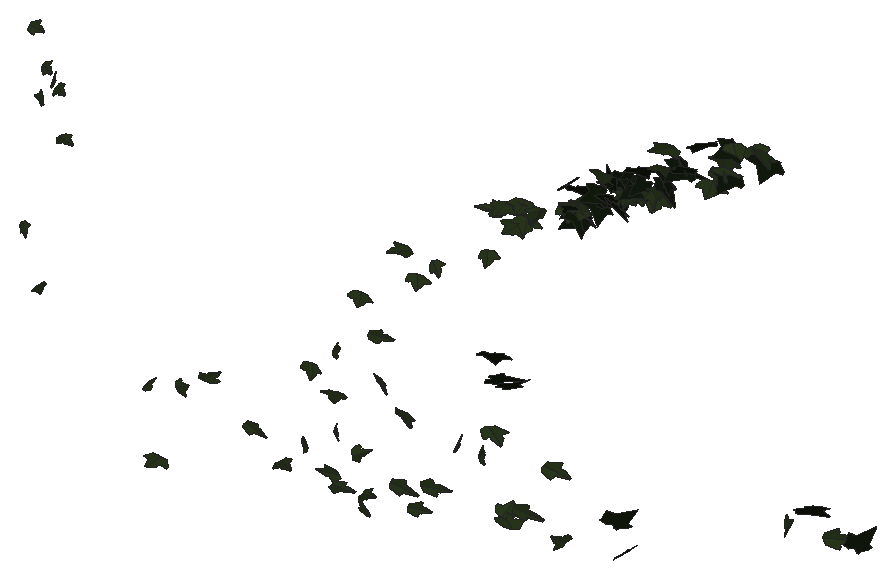
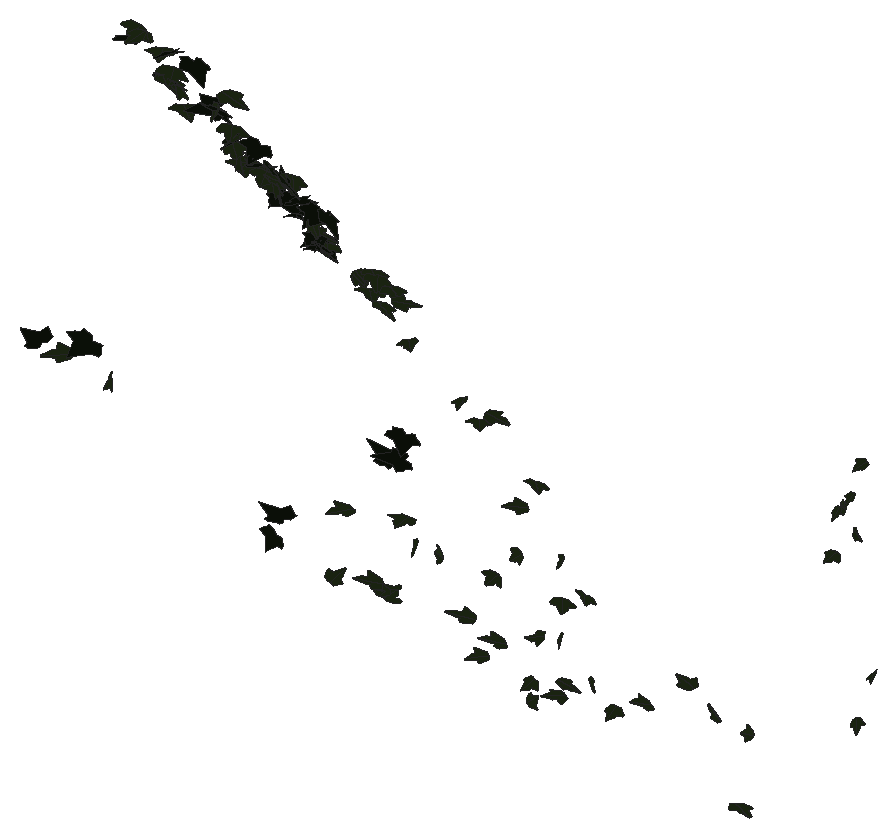
# SketchUp Ruby script. Lengths in millimetres.
U = 1.mm
M = Sketchup.active_model
def pt(a) = Geom::Point3d.new(a.map { |v| v * U })
def face(e, loops, mat)
  f = e.add_face(loops[0].map { |a| pt(a) })
  loops[1..].each { |l| e.add_face(l.map { |a| pt(a) }).erase! }
  f.material = f.back_material = mat if mat
  f
end
# faces: each face lists its corners as indices into pts; further lists are holes
def faces(e, pts, list, mat = nil) = list.each { |f| face(e, (f[0].is_a?(Array) ? f : [f]).map { |l| l.map { |i| pts[i] } }, mat) }
# xy, xz, yz: faces in a plane at the given z, y or x. An outline is a flat list of corners, or four numbers for a rectangle; further outlines are holes
def ring(l) = l.size == 4 ? [[l[0], l[1]], [l[2], l[1]], [l[2], l[3]], [l[0], l[3]]] : l.each_slice(2).to_a
def flat(e, list, mat, &to3) = list.each { |f| face(e, (f[0].is_a?(Array) ? f : [f]).map { |l| ring(l).map { |u, v| to3.(u, v) } }, mat) }
def xy(e, z, list, mat = nil) = flat(e, list, mat) { |x, y| [x, y, z] }
def xz(e, y, list, mat = nil) = flat(e, list, mat) { |x, z| [x, y, z] }
def yz(e, x, list, mat = nil) = flat(e, list, mat) { |y, z| [x, y, z] }
def lines(e, pts, list) = list.each { |a, b| e.add_line(pt(pts[a]), pt(pts[b])) }
# prism: a flat outline (further loops are holes) pulled along v
def prism(e, loops, v, mat = nil)
  f = face(e, loops, mat); d = Geom::Vector3d.new(v.map { |x| x * U })
  f.pushpull(f.normal.samedirection?(d) ? d.length : -d.length)
end
def box(e, o, s, mat = nil) = prism(e, [[o, [o[0] + s[0], o[1], o[2]], [o[0] + s[0], o[1] + s[1], o[2]], [o[0], o[1] + s[1], o[2]]]], [0, 0, s[2]], mat)
def at(x, y, z, deg = 0) = Geom::Transformation.translation(pt([x, y, z])) * Geom::Transformation.rotation(ORIGIN, Z_AXIS, deg.degrees)
def axes(o, x, y, z) = Geom::Transformation.new([*x, 0, *y, 0, *z, 0, *pt(o).to_a, 1])
def part(name) = M.definitions.add(name)
# library, detail: a bought-in or finely detailed component or shape, given as its bounding box
def library(name, o, s) = part(name).tap { |d| box(d.entities, o, s) }
def detail(e, o, s) = box(e.add_group.entities, o, s)
def put(e, d, t, mat = nil) = e.add_instance(d, t).tap { |i| i.material = mat if mat }
def group(e, t, mat = nil) = e.add_group.tap { |g| g.transformation = t; g.material = mat if mat }.entities
root = M.entities
M.materials.add("efeu1").color = [18, 25, 13]
M.materials.add("efeu2").color = [43, 57, 29]
c1 = part("ivyleaf_10")
p = [[0,12.8,-0.8],[-1.5,51.3,-10.9],[-4.9,51,-11.6],[-13.6,26.5,-7.3],[-13.2,15.9,-4.6],[-21.1,19.3,-7.2],
  [-29.5,16.3,-8.3],[-29.2,8.3,-6.2],[-19.7,-9.8,0.5],[-7.6,-13,4],[1,-12.2,5.8],[-0.4,51.1,-11.1],
  [-1.5,51.1,-10.9],[1,-12.4,5.9],[16.9,-12.4,3.5],[35.1,9.1,-5.1],[35,12.9,-6.1],[20.5,16.4,-4.9],
  [15.8,15,-3.8],[15.3,27.6,-7.1],[12.8,31.3,-7.8]]
faces(c1.entities,p,[[0,1,2,3,4,5,6,7,8,9,10],[11,12,0,13,14,15,16,17,18,19,20]],"efeu2")
c2 = part("ivyleaf_9")
p = [[39.1,54.8,31.7],[34.5,51.8,30.2],[-5.3,25.2,17.3],[-17.9,28.3,20.9],[-21.6,21.7,17],[-20.2,4.3,5.3],
  [-22.9,-0.3,2.5],[-17.1,-4,-0.6],[-2,-2.1,-1.2],[-0.7,-15.4,-10.1],[16.6,-22.3,-16.7],[21.1,-15.1,-12.5],
  [32.7,-10.7,-11],[46.1,-1.8,-6.6],[30.8,11.2,3.8]]
faces(c2.entities,p,[[0,1,2,3,4,5,6,7,8,9,10,11,12,13,14]],"efeu1")
put(root,c1,axes([1835,1080.9,259.8],[0.07,0.0363,-0.75049],[0.72421,0.647,0.04994],[1.23306,-0.38207,0.01327]))
put(root,c1,axes([716.7,1092.8,545.6],[-0.03211,0.64084,-0.00687],[0.00479,-0.00671,-0.64137],[-0.78186,-0.02636,-0.00365]))
put(root,c1,axes([1134.4,1084.8,213.7],[0.18479,-0.3198,0.55072],[-0.13417,0.54826,0.3308],[-1.20458,-0.11013,0.04764]))
put(root,c1,axes([755.1,1084.5,1157.1],[0.17773,0.33378,0.55382],[0.19747,0.5308,-0.36249],[-0.76376,0.21491,0.03515]))
put(root,c1,axes([772,1093.8,384.4],[-0.22942,-0.59673,-0.12491],[0.01796,0.12623,-0.62522],[0.74357,-0.18716,-0.02343]))
put(root,c1,axes([850,1090.9,855.9],[-0.51761,-0.26028,-0.40786],[0.44142,0.18947,-0.49728],[0.3919,-0.55719,0.02142]))
put(root,c1,axes([815.9,1090.9,1003.2],[0.31464,-0.47607,0.34173],[-0.21038,0.29518,0.54136],[-0.68329,-0.3101,-0.00932]))
put(root,c1,axes([779.9,1090.9,945],[-0.08194,0.1069,0.6259],[-0.73806,0.18038,-0.09572],[-0.23526,-0.60309,0.08231]))
put(root,c1,axes([793.1,1087.6,1049],[0.02924,0.51162,0.38768],[-0.04677,0.3884,-0.5102],[-0.78173,-0.00411,0.04503]))
put(root,c1,axes([2260.2,1098.7,999.9],[0.65638,0.60263,-0.13044],[-0.19629,-0.09097,-0.69297],[-1.15696,0.35733,0.04357]))
put(root,c1,axes([1958.8,1094.8,204.7],[0.29609,0.07308,0.70938],[1.27007,0.2411,-0.17119],[-0.47857,0.68505,-0.01543]))
put(root,c1,axes([1227.7,1103.9,237.8],[0.58443,-0.30845,-0.46453],[0.60756,-0.33756,0.43517],[-0.87012,-0.44287,-0.00815]))
put(root,c1,axes([2065.8,1090.3,238.7],[-0.15506,-0.04365,0.74271],[1.07084,0.48522,0.09024],[-0.92642,0.56817,-0.02]))
put(root,c1,axes([1888.8,1090.1,630.5],[0.22873,0.00111,0.64955],[0.80459,0.50138,-0.07907],[-0.93855,0.43009,0.09051]))
put(root,c1,axes([1833.4,1100.7,725.7],[1.20506,0.07836,-0.00643],[-0.01143,-0.00382,-0.638],[-0.1492,0.6332,-0.00305]))
put(root,c1,axes([2161.9,1090.9,387.6],[0.43544,-0.49458,0.48892],[-0.33564,0.45661,0.54443],[-1.28032,-0.28791,0.02356]))
put(root,c1,axes([832.1,1095.1,997],[-0.12067,-0.54731,-0.31172],[0.27731,0.26326,-0.53435],[0.71664,-0.19403,0.15429]))
put(root,c1,axes([2022.3,1099.8,844.8],[0.99723,0.41506,-0.01188],[-0.01976,-0.00603,-0.66845],[-0.79003,0.52408,0.00172]))
put(root,c1,axes([1157.7,1102.7,-0.6],[1.01432,0.16087,-0.33534],[-0.61084,-0.09718,-0.55671],[-0.3577,0.62214,-0.00025]))
put(root,c2,axes([2278.7,1091.8,709.9],[0.96894,0.53705,-0.1811],[-0.23679,-0.1316,-0.74001],[-1.05235,0.52409,-0.00024]))
put(root,c2,axes([2681.3,1095.3,1297.3],[1.34853,-0.13217,-0.26729],[-0.50396,0.03793,-0.72071],[0.26093,0.75635,-0.01057]))
put(root,c1,axes([1324.2,1097.1,299.3],[-0.61086,-0.43006,0.38361],[0.44145,0.30555,0.53663],[-1.00403,0.396,0.00255]))
put(root,c1,axes([1578.7,1095.4,139],[-0.5423,-0.5139,-0.37911],[0.42223,0.30962,-0.58645],[1.13969,-0.35924,0.03688]))
put(root,c1,axes([3165.4,1100.4,1618.4],[-1.49985,0.25492,-0.22503],[0.39022,-0.0969,-0.8278],[-0.51628,-0.81382,0.02807]))
put(root,c1,axes([1749.5,1101.1,402.9],[-1.12343,-0.23675,0.0375],[-0.06558,-0.01482,-0.63599],[0.45147,-0.59129,0.00093]))
put(root,c1,axes([2864.2,1103.2,1524.3],[0.82011,0.30587,-0.61086],[-1.25968,0.00806,-0.46287],[-0.32199,0.74751,0.25495]))
put(root,c2,axes([2319.3,1098.5,624.8],[0.92747,0.59527,-0.0229],[0.02688,0.01804,0.7693],[1.13344,-0.48753,0.0005]))
put(root,c1,axes([1746.8,1100.9,162.2],[0.3893,-0.06424,-0.6006],[-1.0995,0.16432,-0.21433],[0.33562,0.61283,-0.00548]))
put(root,c2,axes([3330.2,1087,617.3],[1.21286,0.57336,0.31985],[0.44231,0.21988,-0.85721],[-1.16862,0.67829,0.00751]))
put(root,c1,axes([1891.6,1104.2,494.7],[-0.79385,0.48435,-0.28142],[0.34691,-0.21441,-0.6392],[-1.00809,-0.4552,0.00164]))
put(root,c2,axes([2979,1097.4,1579.8],[0.19677,0.7596,-0.27697],[-0.16077,-0.26755,-0.76529],[-1.53035,0.12577,0.04479]))
put(root,c2,axes([3495.2,1090.6,562.5],[-0.38146,-0.14482,0.9022],[1.41128,0.51393,0.24723],[-1.01616,0.76812,0.00468]))
put(root,c1,axes([1663.6,1106.5,450.6],[1.15689,-0.18495,0.17352],[0.31226,-0.05682,-0.63535],[0.36803,0.62959,-0.00637]))
put(root,c1,axes([2245.2,1089.9,393.7],[-0.18723,0.20672,0.71004],[-0.61655,0.63187,-0.22884],[-1.26523,-0.3385,0.00644]))
put(root,c2,axes([3186.2,1116.5,1593.2],[-0.91707,-0.70197,0.06417],[-0.04945,-0.05998,-0.85134],[1.34064,-0.48239,0.01249]))
put(root,c1,axes([1757.9,1094,292.1],[-0.36104,0.3296,0.51373],[-0.51729,0.43607,-0.38014],[-1.04013,-0.33128,0.01074]))
put(root,c2,axes([3066.2,1121.5,1582.5],[-0.81268,-0.41233,0.56307],[-0.59755,-0.47604,-0.5867],[1.18624,-0.52228,0.09022]))
put(root,c2,axes([2629.2,1120.1,1296.5],[-0.82056,-0.40163,0.52611],[-0.73852,-0.35528,-0.58922],[1.02051,-0.58005,-0.00338]))
put(root,c1,axes([2330.3,1105.3,214.2],[1.22161,0.264,0.30917],[-0.54691,-0.11409,0.69403],[0.54732,-0.70325,0.00347]))
put(root,c2,axes([3060.3,1115.4,1509.6],[-1.47464,-0.18215,-0.25497],[0.51451,-0.04472,-0.78959],[0.30154,-0.81447,0.10037]))
put(root,c1,axes([2498.2,1119.5,213.9],[-0.43074,-0.39702,-0.64952],[-0.61961,-0.56204,0.45699],[-1.30963,0.39649,-0.00258]))
put(root,c1,axes([1458.8,1106.5,200.9],[0.47718,-0.00362,0.59161],[1.11,0.10933,-0.24651],[-0.18894,0.63317,0.04594]))
put(root,c2,axes([2616,1118.7,1265.3],[-0.50362,-0.7383,0.0523],[0.05061,-0.06499,-0.78289],[1.40774,-0.26179,0.04686]))
put(root,c2,axes([2282.3,1095,636.9],[0.2917,0.46147,-0.58792],[0.38466,0.5522,0.48612],[1.36945,-0.2534,-0.01132]))
put(root,c1,axes([3409.6,1091.7,555.7],[0.03177,0.07725,0.92151],[0.62903,0.86028,-0.0781],[-1.64371,0.33071,-0.01208]))
put(root,c2,axes([2755.7,1120.4,1359.4],[-1.20594,-0.37236,0.2477],[-0.29857,-0.21719,-0.72782],[0.79705,-0.64473,0.10213]))
put(root,c2,axes([2908.4,1114.5,1476.5],[-1.56799,-0.06194,-0.06901],[0.12971,0.01391,-0.82615],[0.11967,-0.82664,-0.00873]))
put(root,c2,axes([2833.5,1123,1417.4],[0.0395,-0.59408,0.51555],[0.04397,-0.51504,-0.59443],[1.49639,0.03082,0.00386]))
put(root,c2,axes([2897.7,1099.4,1472.3],[1.25785,0.17443,0.45446],[0.84069,0.10709,-0.6835],[-0.38928,0.7949,-0.00764]))
put(root,c1,axes([2266.2,1105.6,470.5],[0.97995,0.46528,0.31846],[0.45198,0.21218,-0.69398],[-0.97326,0.56702,-0.00163]))
put(root,c1,axes([3017.1,1116,1499.3],[1.27904,-0.44105,0.22768],[0.39036,-0.10222,-0.80342],[0.86023,0.70216,0.02606]))
put(root,c1,axes([3259.4,1094.3,535.3],[0.01905,-0.12864,-0.89619],[0.08006,0.89534,-0.12804],[1.72125,-0.04022,0.01587]))
put(root,c1,axes([1749.7,1105.5,124.9],[-0.40086,-0.11682,-0.592],[1.04087,0.22799,-0.23957],[0.48526,-0.58553,0.02483]))
put(root,c1,axes([3054.6,1113.6,1510],[1.49219,-0.04348,-0.28572],[-0.54339,0.01153,-0.78524],[0.08527,0.8344,-0.00403]))
put(root,c1,axes([2463.3,1102.1,428.4],[0.44702,0.3399,0.67518],[0.77419,0.53909,-0.4129],[-1.21258,0.4695,-0.01471]))
put(root,c1,axes([2742.6,1114.5,1357.5],[1.3846,0.02287,0.33345],[0.63214,0.03971,-0.72739],[-0.07103,0.7993,0.0266]))
put(root,c2,axes([2709.3,1096.8,260.9],[0.40315,0.63216,0.47257],[0.29437,0.44656,-0.6667],[-1.47302,0.26226,-0.0039]))
put(root,c2,axes([2760.9,1122.9,1380.1],[-1.37428,-0.00151,-0.28626],[0.52288,-0.22191,-0.69184],[-0.15309,-0.74439,0.20683]))
put(root,c1,axes([1748.5,1101.6,527.3],[-0.0552,0.13804,0.62277],[-0.43514,0.57975,-0.13915],[-1.13337,-0.22931,0.02309]))
put(root,c1,axes([2832.1,1116.2,1388.5],[-0.81019,-0.68459,0.09379],[-0.07431,-0.08616,-0.80606],[1.31297,-0.42731,0.01226]))
put(root,c1,axes([2073.5,1110.2,896.6],[0.25372,0.65307,0.13137],[-0.01536,0.13555,-0.66565],[-1.26773,0.12906,0.03436]))
put(root,c1,axes([2008.7,1103.4,149.6],[0.23093,0.12235,0.65875],[0.54946,0.59458,-0.16361],[-1.15072,0.30846,0.05408]))
put(root,c2,axes([2668.5,1116.2,1297],[0.35755,0.37763,-0.67113],[-0.69038,-0.56598,-0.42001],[-1.29283,0.40668,0.03867]))
put(root,c1,axes([1844.9,1105,133],[-0.40527,-0.35171,-0.57583],[0.49724,0.51374,-0.41041],[1.184,-0.33614,-0.02474]))
put(root,c2,axes([2672.2,1103.1,1340.8],[0.05746,-0.03122,0.78694],[-0.11229,0.78521,0.03341],[-1.49467,-0.06019,0.02774]))
put(root,c2,axes([2830.5,1120.8,1402.8],[0.22553,-0.76308,-0.14403],[-0.08144,0.13906,-0.77195],[1.47568,0.1243,-0.02059]))
put(root,c1,axes([2802.1,1121.1,1357.9],[-0.24693,-0.77331,0.17823],[0.35479,-0.20525,-0.75481],[1.46809,-0.08047,0.21239]))
put(root,c1,axes([2310.1,1104.3,239.5],[0.57796,0.44876,-0.52822],[0.49248,0.46159,0.54092],[1.22375,-0.3977,0.03178]))
put(root,c1,axes([3141.4,1112.4,1614.9],[-0.78497,-0.55293,-0.4565],[0.92683,0.17052,-0.64654],[1.00162,-0.59112,0.2405]))
put(root,c1,axes([2362.8,1118.8,1179],[1.22698,0.2788,-0.20265],[-0.37201,-0.05828,-0.70201],[-0.54028,0.67328,0.02314]))
put(root,c1,axes([2301.1,1118.6,1148.7],[1.10376,0.31896,-0.30182],[-0.59397,-0.05235,-0.655],[-0.58792,0.65169,0.09511]))
put(root,c1,axes([2639.3,1114.3,1359.3],[-1.45501,-0.01451,0.16094],[-0.30656,0.00646,-0.76459],[0.02449,-0.78124,-0.00931]))
put(root,c1,axes([3068.9,1115.9,1592.3],[1.08153,0.58383,0.07739],[0.10574,0.05393,-0.81473],[-1.11587,0.57097,-0.00219]))
put(root,c1,axes([2707.4,1118.5,1332.7],[1.44036,-0.14576,-0.01688],[-0.01333,0.05269,-0.76907],[0.27894,0.75516,0.0504]))
put(root,c1,axes([1846,1112.5,74.9],[-0.73073,0.39142,-0.35892],[-0.46941,0.26082,0.54827],[0.89512,0.45631,-0.00549]))
put(root,c1,axes([2561.2,1117.6,1228.5],[0.32835,-0.04008,-0.75614],[-1.42615,0.10242,-0.17641],[0.20711,0.76878,-0.01592]))
put(root,c2,axes([2717.6,1115.4,1372.4],[-1.01184,0.55634,-0.04476],[0.05604,-0.03377,-0.76952],[-1.06076,-0.53247,0.00204]))
put(root,c1,axes([2799.4,1119.6,1348.4],[1.49265,0.1598,-0.01715],[-0.02627,-0.01817,-0.80026],[-0.30476,0.78426,-0.01505]))
put(root,c1,axes([2275.2,1125.5,1122.5],[0.02636,0.07794,0.72358],[-0.98559,-0.50742,0.06457],[0.97316,-0.51602,0.0458]))
put(root,c1,axes([1961.5,1117.1,410.7],[-1.15231,0.31636,-0.20066],[0.32986,-0.10155,-0.68307],[-0.63211,-0.62971,0.00934]))
put(root,c1,axes([2893.2,1113.3,1483.4],[-0.81784,0.65069,0.14845],[-0.18624,0.11322,-0.77955],[-1.25648,-0.44031,0.01892]))
put(root,c1,axes([2689.9,1114.2,1317],[0.52975,-0.63522,-0.39024],[-0.24469,0.36941,-0.69302],[1.39761,0.30545,0.02658]))
put(root,c2,axes([2542.8,1128.3,1200],[-0.35767,-0.74405,-0.04972],[0.0421,0.04569,-0.76735],[1.41861,-0.18895,0.01024]))
put(root,c2,axes([2545.1,1118.8,1221.1],[0.43476,0.41205,-0.61528],[-0.74125,-0.48078,-0.46658],[-1.19866,0.44677,0.06537]))
put(root,c1,axes([2725.7,1117.5,1346.2],[-1.41356,-0.18107,-0.11001],[0.20251,0.02801,-0.76448],[0.34868,-0.75031,-0.00199]))
put(root,c1,axes([2988.2,1120.6,1452.6],[1.29824,0.44243,-0.14411],[-0.325,0.00015,-0.80787],[-0.82378,0.69719,0.09162]))
put(root,c2,axes([2670.9,1112.1,334.2],[-0.3625,-0.10209,0.79318],[1.46904,0.18982,0.20979],[-0.39815,0.79334,0.05188]))
put(root,c1,axes([1964.8,1126.8,894.4],[-0.47642,-0.20862,0.59666],[-0.83317,-0.40569,-0.32551],[0.86774,-0.50407,0.01504]))
put(root,c1,axes([3034.6,1118.9,1543.9],[-1.52436,-0.1323,-0.04872],[0.09716,-0.01019,-0.81159],[0.25011,-0.80236,0.01834]))
put(root,c1,axes([1644.3,1111,204.1],[0.10386,-0.1307,-0.62812],[-0.41423,0.58923,-0.14152],[1.14864,0.22431,0.00576]))
put(root,c2,axes([2671.9,1116.7,1357.4],[-0.77887,0.64709,0.05819],[-0.098,0.03625,-0.76527],[-1.23263,-0.41177,0.02407]))
put(root,c1,axes([2403.2,1127.8,1155.5],[-0.34653,-0.6642,0.23474],[-0.01409,-0.24064,-0.68663],[1.34066,-0.17421,0.05346]))
put(root,c1,axes([2404.4,1130.6,1163.9],[-0.53745,-0.59066,0.38104],[-0.0394,-0.40348,-0.64078],[1.33719,-0.24929,0.13427]))
put(root,c2,axes([2552,1127.1,1197],[-1.45741,0.02598,0.00332],[-0.00538,0.01447,-0.76608],[-0.04955,-0.76564,-0.01436]))
put(root,c1,axes([2349.6,1120.2,1166.3],[-1.38941,-0.1153,0.03776],[-0.07322,0.00156,-0.73905],[0.21899,-0.73101,-0.00754]))
put(root,c1,axes([2511.1,1122.4,1208],[1.31074,0.26199,0.09397],[0.15396,0.05154,-0.7366],[-0.50685,0.69317,0.01925]))
put(root,c2,axes([2747.9,1112.1,1418.2],[1.04593,0.5533,0.00685],[0.02163,-0.00163,-0.77979],[-1.05291,0.5496,-0.00921]))
put(root,c1,axes([2700,1122.2,1318.7],[-1.32793,0.29461,0.11061],[-0.31962,-0.12109,-0.73689],[-0.5065,-0.696,0.17502]))
put(root,c2,axes([2535,1120.2,1227],[1.29992,-0.33314,-0.14426],[-0.22607,0.08537,-0.75954],[0.65289,0.69284,0.02423]))
put(root,c1,axes([2833.9,1121.7,1443.3],[-1.3574,-0.33296,-0.03075],[0.04739,0.01934,-0.78708],[0.63462,-0.71362,-0.00699]))
put(root,c2,axes([2520,1116.6,1293.5],[-0.28545,0.74483,-0.05611],[0.0244,-0.05466,-0.75978],[-1.42137,-0.15052,-0.00177]))
put(root,c2,axes([2546.4,1114.4,1290.8],[1.28706,0.36695,-0.01396],[-0.02416,-0.00588,-0.7694],[-0.69846,0.67638,0.00089]))
put(root,c1,axes([2350,1119.6,256.7],[0.26265,0.01796,0.76106],[1.32184,0.31373,-0.13335],[-0.59324,0.70699,0.03983]))
put(root,c1,axes([2560.3,1127.3,1259.5],[-0.24638,-0.76481,0.07929],[-0.01238,-0.07931,-0.77566],[1.46333,-0.12944,0.00679]))
put(root,c1,axes([2366.9,1126,1125.3],[1.31625,0.28041,-0.0603],[-0.10644,-0.02255,-0.74628],[-0.53541,0.69385,0.00012]))
put(root,c1,axes([2331,1125.1,1094.6],[1.20456,-0.18161,-0.33964],[-0.61813,0.09952,-0.65843],[0.394,0.71136,0.0054]))
